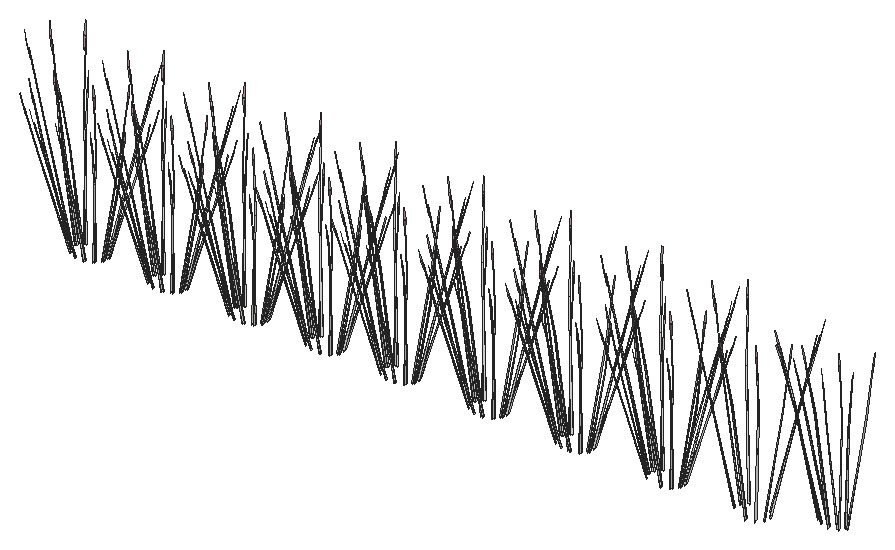
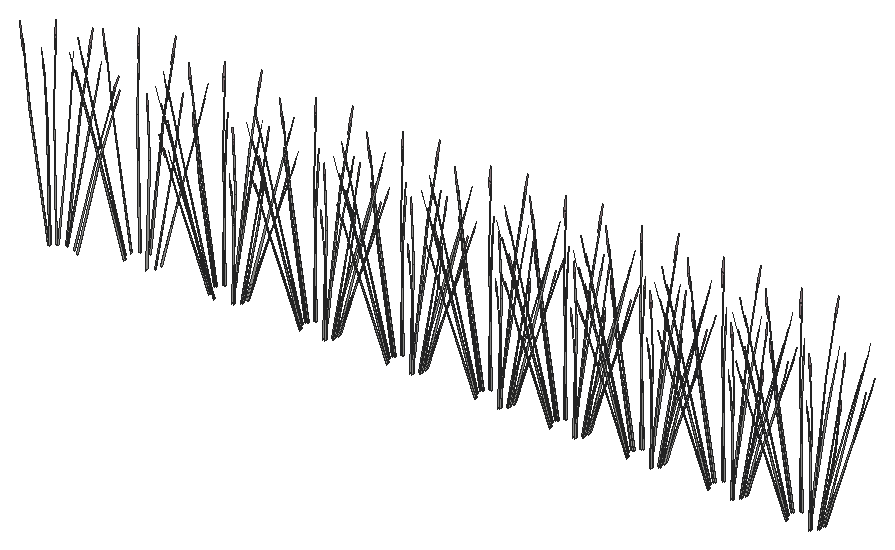
# SketchUp Ruby script. Lengths in inches.
U = 1.inch
M = Sketchup.active_model
def pt(a) = Geom::Point3d.new(a.map { |v| v * U })
def face(e, loops, mat)
  f = e.add_face(loops[0].map { |a| pt(a) })
  loops[1..].each { |l| e.add_face(l.map { |a| pt(a) }).erase! }
  f.material = f.back_material = mat if mat
  f
end
# faces: each face lists its corners as indices into pts; further lists are holes
def faces(e, pts, list, mat = nil) = list.each { |f| face(e, (f[0].is_a?(Array) ? f : [f]).map { |l| l.map { |i| pts[i] } }, mat) }
# xy, xz, yz: faces in a plane at the given z, y or x. An outline is a flat list of corners, or four numbers for a rectangle; further outlines are holes
def ring(l) = l.size == 4 ? [[l[0], l[1]], [l[2], l[1]], [l[2], l[3]], [l[0], l[3]]] : l.each_slice(2).to_a
def flat(e, list, mat, &to3) = list.each { |f| face(e, (f[0].is_a?(Array) ? f : [f]).map { |l| ring(l).map { |u, v| to3.(u, v) } }, mat) }
def xy(e, z, list, mat = nil) = flat(e, list, mat) { |x, y| [x, y, z] }
def xz(e, y, list, mat = nil) = flat(e, list, mat) { |x, z| [x, y, z] }
def yz(e, x, list, mat = nil) = flat(e, list, mat) { |y, z| [x, y, z] }
def lines(e, pts, list) = list.each { |a, b| e.add_line(pt(pts[a]), pt(pts[b])) }
# prism: a flat outline (further loops are holes) pulled along v
def prism(e, loops, v, mat = nil)
  f = face(e, loops, mat); d = Geom::Vector3d.new(v.map { |x| x * U })
  f.pushpull(f.normal.samedirection?(d) ? d.length : -d.length)
end
def box(e, o, s, mat = nil) = prism(e, [[o, [o[0] + s[0], o[1], o[2]], [o[0] + s[0], o[1] + s[1], o[2]], [o[0], o[1] + s[1], o[2]]]], [0, 0, s[2]], mat)
def at(x, y, z, deg = 0) = Geom::Transformation.translation(pt([x, y, z])) * Geom::Transformation.rotation(ORIGIN, Z_AXIS, deg.degrees)
def axes(o, x, y, z) = Geom::Transformation.new([*x, 0, *y, 0, *z, 0, *pt(o).to_a, 1])
def part(name) = M.definitions.add(name)
# library, detail: a bought-in or finely detailed component or shape, given as its bounding box
def library(name, o, s) = part(name).tap { |d| box(d.entities, o, s) }
def detail(e, o, s) = box(e.add_group.entities, o, s)
def put(e, d, t, mat = nil) = e.add_instance(d, t).tap { |i| i.material = mat if mat }
def group(e, t, mat = nil) = e.add_group.tap { |g| g.transformation = t; g.material = mat if mat }.entities
root = M.entities
M.materials.add("LightPink_Translucent").color = [144, 107, 117]
M.materials["LightPink_Translucent"].alpha = 0.75
c1 = part("blade")
p = [[2.15,0.21,22],[0,0.17,0],[0.09,0.45,0],[2.18,0.31,22],[2.29,0.31,22],[0.38,0.45,0],
  [2.48,0.24,33],[2.49,0.24,33],[2.48,0.22,33]]
faces(c1.entities,p,[[0,1,2,3],[4,5,2,3],[6,3,4,7],[8,0,3,6]])
c2 = part("seeds")
p = [[0.3,-0.1,1.38],[-0.01,-0.03,1.59],[-0.01,-0.03,0.03],[0.14,-0.07,-0.07],[0.29,-0.03,3],[0.15,0.01,3.11]]
faces(c2.entities,p,[[0,1,2,3],[1,0,4,5]],"LightPink_Translucent")
c3 = part("blade with seeds")
put(c3.entities,c1,at(0,0,0))
put(c3.entities,c2,axes([2.4,0.25,30.99],[1.5799,-0.05474,1.17369],[-0.12525,1.92788,0.29478],[-0.07173,-0.02425,1.56792]))
put(root,c3,axes([382.81,50.98,259.73],[0.74868,0.15974,0.48003],[-0.25601,0.52518,0.3958],[-0.04499,-0.20653,0.9933]))
put(root,c3,axes([365.17,50.98,259.73],[0.74868,0.15974,0.48003],[-0.25601,0.52518,0.3958],[-0.04499,-0.20653,0.9933]))
put(root,c3,axes([346.39,50.98,259.73],[0.74868,0.15974,0.48003],[-0.25601,0.52518,0.3958],[-0.04499,-0.20653,0.9933]))
put(root,c3,axes([328.48,50.98,259.73],[0.74868,0.15974,0.48003],[-0.25601,0.52518,0.3958],[-0.04499,-0.20653,0.9933]))
put(root,c3,axes([310.38,50.98,259.73],[0.74868,0.15974,0.48003],[-0.25601,0.52518,0.3958],[-0.04499,-0.20653,0.9933]))
put(root,c3,axes([294.93,50.98,259.73],[0.74868,0.15974,0.48003],[-0.25601,0.52518,0.3958],[-0.04499,-0.20653,0.9933]))
put(root,c3,axes([279.2,50.98,259.73],[0.74868,0.15974,0.48003],[-0.25601,0.52518,0.3958],[-0.04499,-0.20653,0.9933]))
put(root,c3,axes([262.47,50.98,259.73],[0.74868,0.15974,0.48003],[-0.25601,0.52518,0.3958],[-0.04499,-0.20653,0.9933]))
put(root,c3,axes([246.41,50.98,259.73],[0.74868,0.15974,0.48003],[-0.25601,0.52518,0.3958],[-0.04499,-0.20653,0.9933]))
put(root,c3,axes([365.37,50.94,259.73],[0.55987,-0.20767,0.0643],[0.27403,0.37869,0.50621],[-0.05407,-0.16693,0.77189]))
put(root,c3,axes([346.59,50.94,259.73],[0.55987,-0.20767,0.0643],[0.27403,0.37869,0.50621],[-0.05407,-0.16693,0.77189]))
put(root,c3,axes([328.68,50.94,259.73],[0.55987,-0.20767,0.0643],[0.27403,0.37869,0.50621],[-0.05407,-0.16693,0.77189]))
put(root,c3,axes([310.58,50.94,259.73],[0.55987,-0.20767,0.0643],[0.27403,0.37869,0.50621],[-0.05407,-0.16693,0.77189]))
put(root,c3,axes([295.13,50.94,259.73],[0.55987,-0.20767,0.0643],[0.27403,0.37869,0.50621],[-0.05407,-0.16693,0.77189]))
put(root,c3,axes([279.4,50.94,259.73],[0.55987,-0.20767,0.0643],[0.27403,0.37869,0.50621],[-0.05407,-0.16693,0.77189]))
put(root,c3,axes([262.67,50.94,259.73],[0.55987,-0.20767,0.0643],[0.27403,0.37869,0.50621],[-0.05407,-0.16693,0.77189]))
put(root,c3,axes([246.61,50.94,259.73],[0.55987,-0.20767,0.0643],[0.27403,0.37869,0.50621],[-0.05407,-0.16693,0.77189]))
put(root,c3,axes([344.67,50.99,259.73],[0.34533,-0.38816,0.0643],[0.49176,0.22599,0.50621],[-0.15898,-0.12445,0.77189]))
put(root,c3,axes([326.77,50.99,259.73],[0.34533,-0.38816,0.0643],[0.49176,0.22599,0.50621],[-0.15898,-0.12445,0.77189]))
put(root,c3,axes([308.66,50.99,259.73],[0.34533,-0.38816,0.0643],[0.49176,0.22599,0.50621],[-0.15898,-0.12445,0.77189]))
put(root,c3,axes([293.21,50.99,259.73],[0.34533,-0.38816,0.0643],[0.49176,0.22599,0.50621],[-0.15898,-0.12445,0.77189]))
put(root,c3,axes([277.48,50.99,259.73],[0.34533,-0.38816,0.0643],[0.49176,0.22599,0.50621],[-0.15898,-0.12445,0.77189]))
put(root,c3,axes([260.75,50.99,259.73],[0.34533,-0.38816,0.0643],[0.49176,0.22599,0.50621],[-0.15898,-0.12445,0.77189]))
put(root,c3,axes([244.6875,50.99,259.73],[0.34533,-0.38816,0.0643],[0.49176,0.22599,0.50621],[-0.15898,-0.12445,0.77189]))
put(root,c3,axes([384.51,51.56,259.73],[0.54105,0.41691,0.48003],[-0.57458,0.35956,0.3958],[0.0998,-0.1956,0.9933]))
put(root,c3,axes([366.875,51.56,259.73],[0.54105,0.41691,0.48003],[-0.57458,0.35956,0.3958],[0.0998,-0.1956,0.9933]))
put(root,c3,axes([348.09,51.56,259.73],[0.54105,0.41691,0.48003],[-0.57458,0.35956,0.3958],[0.0998,-0.1956,0.9933]))
put(root,c3,axes([330.18,51.56,259.73],[0.54105,0.41691,0.48003],[-0.57458,0.35956,0.3958],[0.0998,-0.1956,0.9933]))
put(root,c3,axes([312.08,51.56,259.73],[0.54105,0.41691,0.48003],[-0.57458,0.35956,0.3958],[0.0998,-0.1956,0.9933]))
put(root,c3,axes([296.63,51.56,259.73],[0.54105,0.41691,0.48003],[-0.57458,0.35956,0.3958],[0.0998,-0.1956,0.9933]))
put(root,c3,axes([280.9,51.56,259.73],[0.54105,0.41691,0.48003],[-0.57458,0.35956,0.3958],[0.0998,-0.1956,0.9933]))
put(root,c3,axes([264.17,51.56,259.73],[0.54105,0.41691,0.48003],[-0.57458,0.35956,0.3958],[0.0998,-0.1956,0.9933]))
put(root,c3,axes([248.11,51.56,259.73],[0.54105,0.41691,0.48003],[-0.57458,0.35956,0.3958],[0.0998,-0.1956,0.9933]))
put(root,c3,axes([367.07,51.6,259.73],[0.62439,0.02847,0.0643],[-0.01712,0.42991,0.50621],[0.06534,-0.16468,0.77189]))
put(root,c3,axes([348.29,51.6,259.73],[0.62439,0.02847,0.0643],[-0.01712,0.42991,0.50621],[0.06534,-0.16468,0.77189]))
put(root,c3,axes([330.38,51.6,259.73],[0.62439,0.02847,0.0643],[-0.01712,0.42991,0.50621],[0.06534,-0.16468,0.77189]))
put(root,c3,axes([312.28,51.6,259.73],[0.62439,0.02847,0.0643],[-0.01712,0.42991,0.50621],[0.06534,-0.16468,0.77189]))
put(root,c3,axes([296.83,51.6,259.73],[0.62439,0.02847,0.0643],[-0.01712,0.42991,0.50621],[0.06534,-0.16468,0.77189]))
put(root,c3,axes([281.1,51.6,259.73],[0.62439,0.02847,0.0643],[-0.01712,0.42991,0.50621],[0.06534,-0.16468,0.77189]))
put(root,c3,axes([264.37,51.6,259.73],[0.62439,0.02847,0.0643],[-0.01712,0.42991,0.50621],[0.06534,-0.16468,0.77189]))
put(root,c3,axes([248.31,51.6,259.73],[0.62439,0.02847,0.0643],[-0.01712,0.42991,0.50621],[0.06534,-0.16468,0.77189]))
put(root,c3,axes([361.83,51.76,259.73],[0.03826,-0.46465,0.0643],[0.57772,0.01274,0.50621],[-0.2213,-0.04862,0.77189]))
put(root,c3,axes([343.05,51.76,259.73],[0.03826,-0.46465,0.0643],[0.57772,0.01274,0.50621],[-0.2213,-0.04862,0.77189]))
put(root,c3,axes([325.14,51.76,259.73],[0.03826,-0.46465,0.0643],[0.57772,0.01274,0.50621],[-0.2213,-0.04862,0.77189]))
put(root,c3,axes([307.04,51.76,259.73],[0.03826,-0.46465,0.0643],[0.57772,0.01274,0.50621],[-0.2213,-0.04862,0.77189]))
put(root,c3,axes([291.59,51.76,259.73],[0.03826,-0.46465,0.0643],[0.57772,0.01274,0.50621],[-0.2213,-0.04862,0.77189]))
put(root,c3,axes([275.86,51.76,259.73],[0.03826,-0.46465,0.0643],[0.57772,0.01274,0.50621],[-0.2213,-0.04862,0.77189]))
put(root,c3,axes([259.13,51.76,259.73],[0.03826,-0.46465,0.0643],[0.57772,0.01274,0.50621],[-0.2213,-0.04862,0.77189]))
put(root,c3,axes([243.07,51.76,259.73],[0.03826,-0.46465,0.0643],[0.57772,0.01274,0.50621],[-0.2213,-0.04862,0.77189]))
put(root,c3,axes([368.1,52.81,259.73],[0.52161,0.25698,0.0643],[-0.30368,0.36595,0.50621],[0.16723,-0.11831,0.77189]))
put(root,c3,axes([349.32,52.81,259.73],[0.52161,0.25698,0.0643],[-0.30368,0.36595,0.50621],[0.16723,-0.11831,0.77189]))
put(root,c3,axes([331.41,52.81,259.73],[0.52161,0.25698,0.0643],[-0.30368,0.36595,0.50621],[0.16723,-0.11831,0.77189]))
put(root,c3,axes([313.3,52.81,259.73],[0.52161,0.25698,0.0643],[-0.30368,0.36595,0.50621],[0.16723,-0.11831,0.77189]))
put(root,c3,axes([297.85,52.81,259.73],[0.52161,0.25698,0.0643],[-0.30368,0.36595,0.50621],[0.16723,-0.11831,0.77189]))
put(root,c3,axes([282.125,52.81,259.73],[0.52161,0.25698,0.0643],[-0.30368,0.36595,0.50621],[0.16723,-0.11831,0.77189]))
put(root,c3,axes([265.4,52.81,259.73],[0.52161,0.25698,0.0643],[-0.30368,0.36595,0.50621],[0.16723,-0.11831,0.77189]))
put(root,c3,axes([249.33,52.81,259.73],[0.52161,0.25698,0.0643],[-0.30368,0.36595,0.50621],[0.16723,-0.11831,0.77189]))
put(root,c3,axes([385.59,52.7,259.73],[0.18844,0.56237,0.48003],[-0.73919,0.0976,0.3958],[0.21785,-0.13226,0.9933]))
put(root,c3,axes([367.95,52.7,259.73],[0.18844,0.56237,0.48003],[-0.73919,0.0976,0.3958],[0.21785,-0.13226,0.9933]))
put(root,c3,axes([349.17,52.7,259.73],[0.18844,0.56237,0.48003],[-0.73919,0.0976,0.3958],[0.21785,-0.13226,0.9933]))
put(root,c3,axes([331.26,52.7,259.73],[0.18844,0.56237,0.48003],[-0.73919,0.0976,0.3958],[0.21785,-0.13226,0.9933]))
put(root,c3,axes([313.16,52.7,259.73],[0.18844,0.56237,0.48003],[-0.73919,0.0976,0.3958],[0.21785,-0.13226,0.9933]))
put(root,c3,axes([297.71,52.7,259.73],[0.18844,0.56237,0.48003],[-0.73919,0.0976,0.3958],[0.21785,-0.13226,0.9933]))
put(root,c3,axes([281.98,52.7,259.73],[0.18844,0.56237,0.48003],[-0.73919,0.0976,0.3958],[0.21785,-0.13226,0.9933]))
put(root,c3,axes([265.25,52.7,259.73],[0.18844,0.56237,0.48003],[-0.73919,0.0976,0.3958],[0.21785,-0.13226,0.9933]))
put(root,c3,axes([249.1875,52.7,259.73],[0.18844,0.56237,0.48003],[-0.73919,0.0976,0.3958],[0.21785,-0.13226,0.9933]))
put(root,c3,axes([378.63,53.17,259.73],[0.21466,-0.55714,0.48003],[0.70573,0.19051,0.3958],[-0.27753,0.03348,0.9933]))
put(root,c3,axes([360.99,53.17,259.73],[0.21466,-0.55714,0.48003],[0.70573,0.19051,0.3958],[-0.27753,0.03348,0.9933]))
put(root,c3,axes([342.21,53.17,259.73],[0.21466,-0.55714,0.48003],[0.70573,0.19051,0.3958],[-0.27753,0.03348,0.9933]))
put(root,c3,axes([324.31,53.17,259.73],[0.21466,-0.55714,0.48003],[0.70573,0.19051,0.3958],[-0.27753,0.03348,0.9933]))
put(root,c3,axes([306.2,53.17,259.73],[0.21466,-0.55714,0.48003],[0.70573,0.19051,0.3958],[-0.27753,0.03348,0.9933]))
put(root,c3,axes([290.75,53.17,259.73],[0.21466,-0.55714,0.48003],[0.70573,0.19051,0.3958],[-0.27753,0.03348,0.9933]))
put(root,c3,axes([275.02,53.17,259.73],[0.21466,-0.55714,0.48003],[0.70573,0.19051,0.3958],[-0.27753,0.03348,0.9933]))
put(root,c3,axes([258.29,53.17,259.73],[0.21466,-0.55714,0.48003],[0.70573,0.19051,0.3958],[-0.27753,0.03348,0.9933]))
put(root,c3,axes([242.23,53.17,259.73],[0.21466,-0.55714,0.48003],[0.70573,0.19051,0.3958],[-0.27753,0.03348,0.9933]))
put(root,c3,axes([360.94,53.02,259.73],[-0.27906,-0.41663,0.0643],[0.50888,-0.20393,0.50621],[-0.22432,0.04024,0.77189]))
put(root,c3,axes([342.16,53.02,259.73],[-0.27906,-0.41663,0.0643],[0.50888,-0.20393,0.50621],[-0.22432,0.04024,0.77189]))
put(root,c3,axes([324.25,53.02,259.73],[-0.27906,-0.41663,0.0643],[0.50888,-0.20393,0.50621],[-0.22432,0.04024,0.77189]))
put(root,c3,axes([306.14,53.02,259.73],[-0.27906,-0.41663,0.0643],[0.50888,-0.20393,0.50621],[-0.22432,0.04024,0.77189]))
put(root,c3,axes([290.7,53.02,259.73],[-0.27906,-0.41663,0.0643],[0.50888,-0.20393,0.50621],[-0.22432,0.04024,0.77189]))
put(root,c3,axes([274.97,53.02,259.73],[-0.27906,-0.41663,0.0643],[0.50888,-0.20393,0.50621],[-0.22432,0.04024,0.77189]))
put(root,c3,axes([258.24,53.02,259.73],[-0.27906,-0.41663,0.0643],[0.50888,-0.20393,0.50621],[-0.22432,0.04024,0.77189]))
put(root,c3,axes([242.17,53.02,259.73],[-0.27906,-0.41663,0.0643],[0.50888,-0.20393,0.50621],[-0.22432,0.04024,0.77189]))
put(root,c3,axes([394.94,57.2,259.73],[0.74868,0.15974,0.48003],[-0.25601,0.52518,0.3958],[-0.04499,-0.20653,0.9933]))
put(root,c3,axes([368.18,54.23,259.73],[0.27906,0.41663,0.0643],[-0.50888,0.20393,0.50621],[0.22432,-0.04024,0.77189]))
put(root,c3,axes([349.39,54.23,259.73],[0.27906,0.41663,0.0643],[-0.50888,0.20393,0.50621],[0.22432,-0.04024,0.77189]))
put(root,c3,axes([331.49,54.23,259.73],[0.27906,0.41663,0.0643],[-0.50888,0.20393,0.50621],[0.22432,-0.04024,0.77189]))
put(root,c3,axes([313.38,54.23,259.73],[0.27906,0.41663,0.0643],[-0.50888,0.20393,0.50621],[0.22432,-0.04024,0.77189]))
put(root,c3,axes([297.93,54.23,259.73],[0.27906,0.41663,0.0643],[-0.50888,0.20393,0.50621],[0.22432,-0.04024,0.77189]))
put(root,c3,axes([282.2,54.23,259.73],[0.27906,0.41663,0.0643],[-0.50888,0.20393,0.50621],[0.22432,-0.04024,0.77189]))
put(root,c3,axes([265.48,54.23,259.73],[0.27906,0.41663,0.0643],[-0.50888,0.20393,0.50621],[0.22432,-0.04024,0.77189]))
put(root,c3,axes([249.41,54.23,259.73],[0.27906,0.41663,0.0643],[-0.50888,0.20393,0.50621],[0.22432,-0.04024,0.77189]))
put(root,c3,axes([385.76,54.09,259.73],[-0.21466,0.55714,0.48003],[-0.70573,-0.19051,0.3958],[0.27753,-0.03348,0.9933]))
put(root,c3,axes([368.125,54.09,259.73],[-0.21466,0.55714,0.48003],[-0.70573,-0.19051,0.3958],[0.27753,-0.03348,0.9933]))
put(root,c3,axes([349.34,54.09,259.73],[-0.21466,0.55714,0.48003],[-0.70573,-0.19051,0.3958],[0.27753,-0.03348,0.9933]))
put(root,c3,axes([331.43,54.09,259.73],[-0.21466,0.55714,0.48003],[-0.70573,-0.19051,0.3958],[0.27753,-0.03348,0.9933]))
put(root,c3,axes([313.33,54.09,259.73],[-0.21466,0.55714,0.48003],[-0.70573,-0.19051,0.3958],[0.27753,-0.03348,0.9933]))
put(root,c3,axes([297.88,54.09,259.73],[-0.21466,0.55714,0.48003],[-0.70573,-0.19051,0.3958],[0.27753,-0.03348,0.9933]))
put(root,c3,axes([282.15,54.09,259.73],[-0.21466,0.55714,0.48003],[-0.70573,-0.19051,0.3958],[0.27753,-0.03348,0.9933]))
put(root,c3,axes([265.42,54.09,259.73],[-0.21466,0.55714,0.48003],[-0.70573,-0.19051,0.3958],[0.27753,-0.03348,0.9933]))
put(root,c3,axes([249.36,54.09,259.73],[-0.21466,0.55714,0.48003],[-0.70573,-0.19051,0.3958],[0.27753,-0.03348,0.9933]))
put(root,c3,axes([394.93,57.59,260.05],[-0.22906,0.4699,0.35414],[-0.66828,-0.13705,-0.4572],[-0.06128,-0.18919,0.87481]))
put(root,c3,axes([396.64,57.79,259.73],[0.54105,0.41691,0.48003],[-0.57458,0.35956,0.3958],[0.0998,-0.1956,0.9933]))
put(root,c3,axes([396.375,58.12,260.05],[-0.5141,0.32171,0.35414],[-0.48666,-0.36734,-0.4572],[0.07405,-0.18664,0.87481]))
put(root,c3,axes([393.33,57.67,260.05],[0.11735,0.49217,0.35414],[-0.67083,0.12996,-0.4572],[-0.18018,-0.14104,0.87481]))
put(root,c3,axes([378.8,54.56,259.73],[-0.18844,-0.56237,0.48003],[0.73919,-0.0976,0.3958],[-0.21785,0.13226,0.9933]))
put(root,c3,axes([361.16,54.56,259.73],[-0.18844,-0.56237,0.48003],[0.73919,-0.0976,0.3958],[-0.21785,0.13226,0.9933]))
put(root,c3,axes([342.38,54.56,259.73],[-0.18844,-0.56237,0.48003],[0.73919,-0.0976,0.3958],[-0.21785,0.13226,0.9933]))
put(root,c3,axes([324.48,54.56,259.73],[-0.18844,-0.56237,0.48003],[0.73919,-0.0976,0.3958],[-0.21785,0.13226,0.9933]))
put(root,c3,axes([306.37,54.56,259.73],[-0.18844,-0.56237,0.48003],[0.73919,-0.0976,0.3958],[-0.21785,0.13226,0.9933]))
put(root,c3,axes([290.92,54.56,259.73],[-0.18844,-0.56237,0.48003],[0.73919,-0.0976,0.3958],[-0.21785,0.13226,0.9933]))
put(root,c3,axes([275.19,54.56,259.73],[-0.18844,-0.56237,0.48003],[0.73919,-0.0976,0.3958],[-0.21785,0.13226,0.9933]))
put(root,c3,axes([258.46,54.56,259.73],[-0.18844,-0.56237,0.48003],[0.73919,-0.0976,0.3958],[-0.21785,0.13226,0.9933]))
put(root,c3,axes([242.4,54.56,259.73],[-0.18844,-0.56237,0.48003],[0.73919,-0.0976,0.3958],[-0.21785,0.13226,0.9933]))
put(root,c3,axes([361.02,54.45,259.73],[-0.52161,-0.25698,0.0643],[0.30368,-0.36595,0.50621],[-0.16723,0.11831,0.77189]))
put(root,c3,axes([342.24,54.45,259.73],[-0.52161,-0.25698,0.0643],[0.30368,-0.36595,0.50621],[-0.16723,0.11831,0.77189]))
put(root,c3,axes([324.33,54.45,259.73],[-0.52161,-0.25698,0.0643],[0.30368,-0.36595,0.50621],[-0.16723,0.11831,0.77189]))
put(root,c3,axes([306.22,54.45,259.73],[-0.52161,-0.25698,0.0643],[0.30368,-0.36595,0.50621],[-0.16723,0.11831,0.77189]))
put(root,c3,axes([290.77,54.45,259.73],[-0.52161,-0.25698,0.0643],[0.30368,-0.36595,0.50621],[-0.16723,0.11831,0.77189]))
put(root,c3,axes([275.05,54.45,259.73],[-0.52161,-0.25698,0.0643],[0.30368,-0.36595,0.50621],[-0.16723,0.11831,0.77189]))
put(root,c3,axes([258.32,54.45,259.73],[-0.52161,-0.25698,0.0643],[0.30368,-0.36595,0.50621],[-0.16723,0.11831,0.77189]))
put(root,c3,axes([242.25,54.45,259.73],[-0.52161,-0.25698,0.0643],[0.30368,-0.36595,0.50621],[-0.16723,0.11831,0.77189]))
put(root,c3,axes([397.27,59.11,260.05],[-0.66138,0.08733,0.35414],[-0.17464,-0.49921,-0.4572],[0.18953,-0.13408,0.87481]))
put(root,c3,axes([367.29,55.5,259.73],[-0.03826,0.46465,0.0643],[-0.57772,-0.01274,0.50621],[0.2213,0.04862,0.77189]))
put(root,c3,axes([348.5,55.5,259.73],[-0.03826,0.46465,0.0643],[-0.57772,-0.01274,0.50621],[0.2213,0.04862,0.77189]))
put(root,c3,axes([330.6,55.5,259.73],[-0.03826,0.46465,0.0643],[-0.57772,-0.01274,0.50621],[0.2213,0.04862,0.77189]))
put(root,c3,axes([312.49,55.5,259.73],[-0.03826,0.46465,0.0643],[-0.57772,-0.01274,0.50621],[0.2213,0.04862,0.77189]))
put(root,c3,axes([297.04,55.5,259.73],[-0.03826,0.46465,0.0643],[-0.57772,-0.01274,0.50621],[0.2213,0.04862,0.77189]))
put(root,c3,axes([281.3125,55.5,259.73],[-0.03826,0.46465,0.0643],[-0.57772,-0.01274,0.50621],[0.2213,0.04862,0.77189]))
put(root,c3,axes([264.58,55.5,259.73],[-0.03826,0.46465,0.0643],[-0.57772,-0.01274,0.50621],[0.2213,0.04862,0.77189]))
put(root,c3,axes([248.52,55.5,259.73],[-0.03826,0.46465,0.0643],[-0.57772,-0.01274,0.50621],[0.2213,0.04862,0.77189]))
put(root,c3,axes([384.97,55.35,259.73],[-0.56024,0.40262,0.48003],[-0.48318,-0.42758,0.3958],[0.26285,0.07427,0.9933]))
put(root,c3,axes([367.34,55.35,259.73],[-0.56024,0.40262,0.48003],[-0.48318,-0.42758,0.3958],[0.26285,0.07427,0.9933]))
put(root,c3,axes([348.56,55.35,259.73],[-0.56024,0.40262,0.48003],[-0.48318,-0.42758,0.3958],[0.26285,0.07427,0.9933]))
put(root,c3,axes([330.65,55.35,259.73],[-0.56024,0.40262,0.48003],[-0.48318,-0.42758,0.3958],[0.26285,0.07427,0.9933]))
put(root,c3,axes([312.54,55.35,259.73],[-0.56024,0.40262,0.48003],[-0.48318,-0.42758,0.3958],[0.26285,0.07427,0.9933]))
put(root,c3,axes([297.09,55.35,259.73],[-0.56024,0.40262,0.48003],[-0.48318,-0.42758,0.3958],[0.26285,0.07427,0.9933]))
put(root,c3,axes([281.37,55.35,259.73],[-0.56024,0.40262,0.48003],[-0.48318,-0.42758,0.3958],[0.26285,0.07427,0.9933]))
put(root,c3,axes([264.64,55.35,259.73],[-0.56024,0.40262,0.48003],[-0.48318,-0.42758,0.3958],[0.26285,0.07427,0.9933]))
put(root,c3,axes([248.57,55.35,259.73],[-0.56024,0.40262,0.48003],[-0.48318,-0.42758,0.3958],[0.26285,0.07427,0.9933]))
put(root,c3,axes([397.72,58.93,259.73],[0.18844,0.56237,0.48003],[-0.73919,0.0976,0.3958],[0.21785,-0.13226,0.9933]))
put(root,c3,axes([391.99,58.33,260.05],[0.43232,0.38257,0.35414],[-0.49364,0.36215,-0.4572],[-0.25081,-0.0551,0.87481]))
put(root,c3,axes([362.05,55.66,259.73],[-0.62439,-0.02847,0.0643],[0.01712,-0.42991,0.50621],[-0.06534,0.16468,0.77189]))
put(root,c3,axes([343.26,55.66,259.73],[-0.62439,-0.02847,0.0643],[0.01712,-0.42991,0.50621],[-0.06534,0.16468,0.77189]))
put(root,c3,axes([325.36,55.66,259.73],[-0.62439,-0.02847,0.0643],[0.01712,-0.42991,0.50621],[-0.06534,0.16468,0.77189]))
put(root,c3,axes([307.25,55.66,259.73],[-0.62439,-0.02847,0.0643],[0.01712,-0.42991,0.50621],[-0.06534,0.16468,0.77189]))
put(root,c3,axes([291.8,55.66,259.73],[-0.62439,-0.02847,0.0643],[0.01712,-0.42991,0.50621],[-0.06534,0.16468,0.77189]))
put(root,c3,axes([276.07,55.66,259.73],[-0.62439,-0.02847,0.0643],[0.01712,-0.42991,0.50621],[-0.06534,0.16468,0.77189]))
put(root,c3,axes([259.34,55.66,259.73],[-0.62439,-0.02847,0.0643],[0.01712,-0.42991,0.50621],[-0.06534,0.16468,0.77189]))
put(root,c3,axes([243.28,55.66,259.73],[-0.62439,-0.02847,0.0643],[0.01712,-0.42991,0.50621],[-0.06534,0.16468,0.77189]))
put(root,c3,axes([379.88,55.7,259.73],[-0.54105,-0.41691,0.48003],[0.57458,-0.35956,0.3958],[-0.0998,0.1956,0.9933]))
put(root,c3,axes([362.24,55.7,259.73],[-0.54105,-0.41691,0.48003],[0.57458,-0.35956,0.3958],[-0.0998,0.1956,0.9933]))
put(root,c3,axes([343.46,55.7,259.73],[-0.54105,-0.41691,0.48003],[0.57458,-0.35956,0.3958],[-0.0998,0.1956,0.9933]))
put(root,c3,axes([325.56,55.7,259.73],[-0.54105,-0.41691,0.48003],[0.57458,-0.35956,0.3958],[-0.0998,0.1956,0.9933]))
put(root,c3,axes([307.45,55.7,259.73],[-0.54105,-0.41691,0.48003],[0.57458,-0.35956,0.3958],[-0.0998,0.1956,0.9933]))
put(root,c3,axes([292,55.7,259.73],[-0.54105,-0.41691,0.48003],[0.57458,-0.35956,0.3958],[-0.0998,0.1956,0.9933]))
put(root,c3,axes([276.27,55.7,259.73],[-0.54105,-0.41691,0.48003],[0.57458,-0.35956,0.3958],[-0.0998,0.1956,0.9933]))
put(root,c3,axes([259.54,55.7,259.73],[-0.54105,-0.41691,0.48003],[0.57458,-0.35956,0.3958],[-0.0998,0.1956,0.9933]))
put(root,c3,axes([243.48,55.7,259.73],[-0.54105,-0.41691,0.48003],[0.57458,-0.35956,0.3958],[-0.0998,0.1956,0.9933]))
put(root,c3,axes([365.66,56.26,259.73],[-0.34533,0.38816,0.0643],[-0.49176,-0.22599,0.50621],[0.15898,0.12445,0.77189]))
